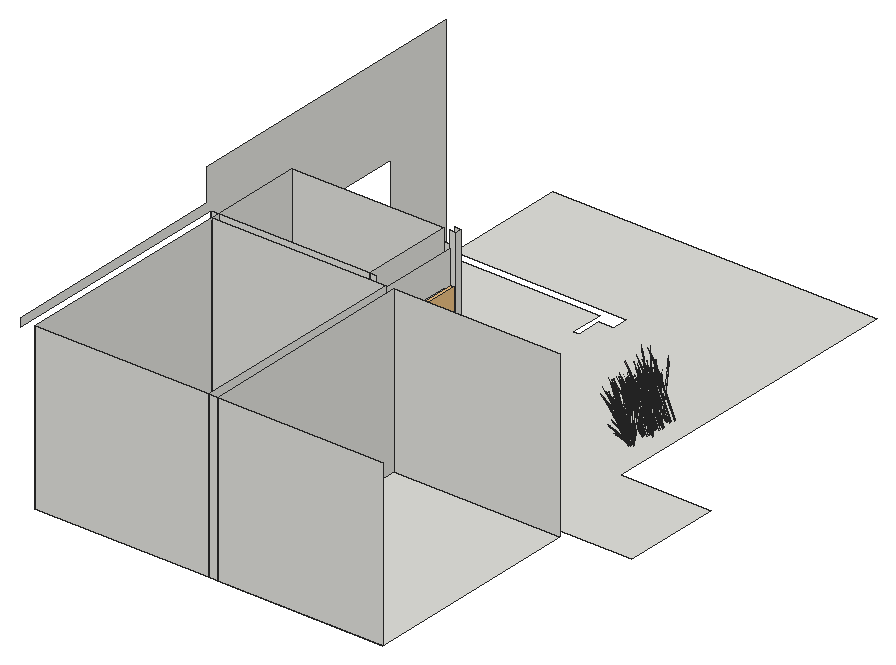
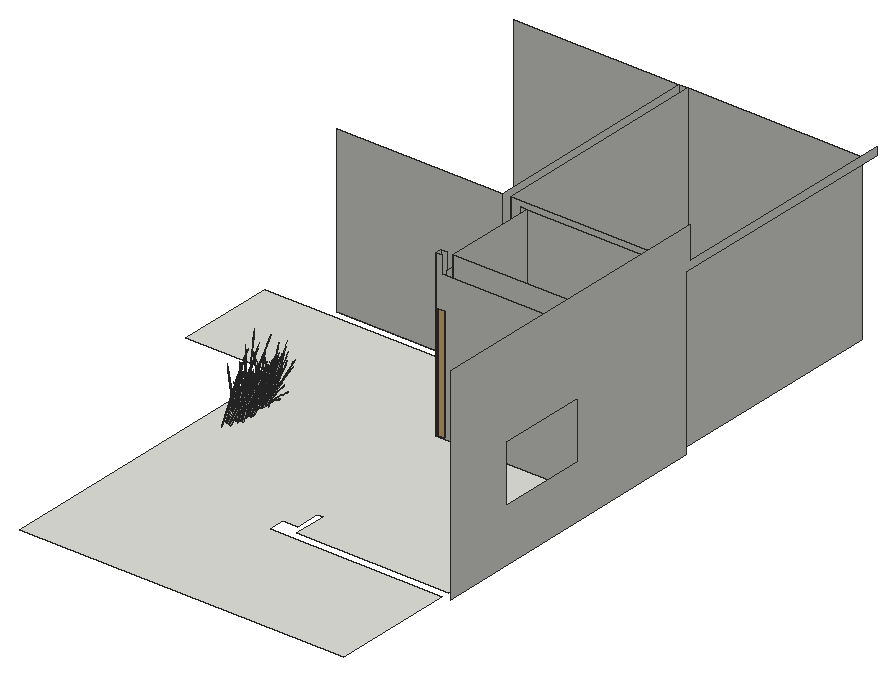
# SketchUp Ruby script. Lengths in inches.
U = 1.inch
M = Sketchup.active_model
def pt(a) = Geom::Point3d.new(a.map { |v| v * U })
def face(e, loops, mat)
  f = e.add_face(loops[0].map { |a| pt(a) })
  loops[1..].each { |l| e.add_face(l.map { |a| pt(a) }).erase! }
  f.material = f.back_material = mat if mat
  f
end
# faces: each face lists its corners as indices into pts; further lists are holes
def faces(e, pts, list, mat = nil) = list.each { |f| face(e, (f[0].is_a?(Array) ? f : [f]).map { |l| l.map { |i| pts[i] } }, mat) }
# xy, xz, yz: faces in a plane at the given z, y or x. An outline is a flat list of corners, or four numbers for a rectangle; further outlines are holes
def ring(l) = l.size == 4 ? [[l[0], l[1]], [l[2], l[1]], [l[2], l[3]], [l[0], l[3]]] : l.each_slice(2).to_a
def flat(e, list, mat, &to3) = list.each { |f| face(e, (f[0].is_a?(Array) ? f : [f]).map { |l| ring(l).map { |u, v| to3.(u, v) } }, mat) }
def xy(e, z, list, mat = nil) = flat(e, list, mat) { |x, y| [x, y, z] }
def xz(e, y, list, mat = nil) = flat(e, list, mat) { |x, z| [x, y, z] }
def yz(e, x, list, mat = nil) = flat(e, list, mat) { |y, z| [x, y, z] }
def lines(e, pts, list) = list.each { |a, b| e.add_line(pt(pts[a]), pt(pts[b])) }
# prism: a flat outline (further loops are holes) pulled along v
def prism(e, loops, v, mat = nil)
  f = face(e, loops, mat); d = Geom::Vector3d.new(v.map { |x| x * U })
  f.pushpull(f.normal.samedirection?(d) ? d.length : -d.length)
end
def box(e, o, s, mat = nil) = prism(e, [[o, [o[0] + s[0], o[1], o[2]], [o[0] + s[0], o[1] + s[1], o[2]], [o[0], o[1] + s[1], o[2]]]], [0, 0, s[2]], mat)
def at(x, y, z, deg = 0) = Geom::Transformation.translation(pt([x, y, z])) * Geom::Transformation.rotation(ORIGIN, Z_AXIS, deg.degrees)
def axes(o, x, y, z) = Geom::Transformation.new([*x, 0, *y, 0, *z, 0, *pt(o).to_a, 1])
def part(name) = M.definitions.add(name)
# library, detail: a bought-in or finely detailed component or shape, given as its bounding box
def library(name, o, s) = part(name).tap { |d| box(d.entities, o, s) }
def detail(e, o, s) = box(e.add_group.entities, o, s)
def put(e, d, t, mat = nil) = e.add_instance(d, t).tap { |i| i.material = mat if mat }
def group(e, t, mat = nil) = e.add_group.tap { |g| g.transformation = t; g.material = mat if mat }.entities
root = M.entities
M.materials.add("LightPink_Translucent").color = [144, 107, 117]
M.materials["LightPink_Translucent"].alpha = 0.75
c1 = library("porta+4",[0.2,-5.42,1.33],[46.55,4.72,83.21])
c2 = part("blade")
p = [[2.15,0.21,22],[0,0.17,0],[0.09,0.45,0],[2.18,0.31,22],[2.29,0.31,22],[0.38,0.45,0],
  [2.48,0.24,33],[2.49,0.24,33],[2.48,0.22,33]]
faces(c2.entities,p,[[0,1,2,3],[4,5,2,3],[6,3,4,7],[8,0,3,6]])
c3 = part("seeds")
p = [[0.3,-0.1,1.38],[-0.01,-0.03,1.59],[-0.01,-0.03,0.03],[0.14,-0.07,-0.07],[0.29,-0.03,3],[0.15,0.01,3.11]]
faces(c3.entities,p,[[0,1,2,3],[1,0,4,5]],"LightPink_Translucent")
c4 = part("blade with seeds")
put(c4.entities,c2,at(0,0,0))
put(c4.entities,c3,axes([2.4,0.25,30.99],[1.5799,-0.05474,1.17369],[-0.12525,1.92788,0.29478],[-0.07173,-0.02425,1.56792]))
xy(root,126,[[51,51,178.5,213],[184.5,51,306,213],[166.5,219,354,219,354,291,288,291,288,525,51,525,51,435,177,435,177,423,166.5,423,166.5,405,162,405,162,429,51,429,51,291,171,291,171,286.5,166.5,286.5],[51,219,162,286.5]])
xz(root,51,[[51,126,178.5,246],[178.5,126,184.5,246],[184.5,126,306,246]])
xz(root,213,[[51,126,178.5,246],[184.5,126,306,246]])
xz(root,219,[[45,126,51,246],[51,126,162,246],[162,126,166.5,246]])
xz(root,286.5,[[51,126,162,246],[166.5,126,171,246]])
xz(root,291,[[51,126,51,234,166.5,234,166.5,246,171,246,171,126]])
yz(root,45,[[[219,126,219,246,45,246,45,252,216,252,216,276,435,276,435,126],[318,165,384,207]]])
yz(root,51,[[51,126,213,246],[213,126,219,246],[219,126,286.5,246]])
yz(root,162,[[[219,126,286.5,246],[247.5,129,277.5,207]]])
yz(root,166.5,[[219,126,244.5,126,244.5,210,280.5,210,280.5,126,286.5,126,286.5,234,219,234],[[244.5,126,280.5,210],[247.5,129,277.5,207]]])
yz(root,171,[[286.5,126,291,246]])
yz(root,178.5,[[51,126,213,246]])
yz(root,184.5,[[51,126,213,246]])
put(root,c1,at(163.74,244.3,125.48,90))
put(root,c4,axes([268.35,323.37,125.98],[0.37107,-0.01478,1.71376],[-0.24616,0.64047,0.13857],[-0.5288,-0.03961,0.73262]))
put(root,c4,axes([268.35,336.34,126.89],[0.37107,-0.01478,1.71376],[-0.24616,0.64047,0.13857],[-0.5288,-0.03961,0.73262]))
put(root,c4,axes([268.35,346.62,126.2],[0.37107,-0.01478,1.71376],[-0.24616,0.64047,0.13857],[-0.5288,-0.03961,0.73262]))
put(root,c4,axes([268.51,324.49,125.98],[0.31041,-0.13801,1.71376],[0.26133,0.63772,0.13857],[-0.48731,0.14413,0.73262]))
put(root,c4,axes([268.51,337.47,126.89],[0.31041,-0.13801,1.71376],[0.26133,0.63772,0.13857],[-0.48731,0.14413,0.73262]))
put(root,c4,axes([268.51,347.75,126.2],[0.31041,-0.13801,1.71376],[0.26133,0.63772,0.13857],[-0.48731,0.14413,0.73262]))
put(root,c4,axes([270.29,336.8,126.35],[0.25429,-0.09438,1.77064],[0.08769,0.65901,0.13857],[-0.5508,0.08745,0.63284]))
put(root,c4,axes([270.29,347.08,125.67],[0.25429,-0.09438,1.77064],[0.08769,0.65901,0.13857],[-0.5508,0.08745,0.63284]))
put(root,c4,axes([267.56,324.27,126.82],[-0.14609,0.08471,1.74944],[0.01243,0.61893,-0.27667],[-0.33486,0.08049,0.14031]))
put(root,c4,axes([267.56,347.52,127.04],[-0.14609,0.08471,1.74944],[0.01243,0.61893,-0.27667],[-0.33486,0.08049,0.14031]))
put(root,c4,axes([269.46,335.75,127.99],[-0.89428,-0.01571,-0.71045],[0.06006,-0.66153,0.08574],[-0.37886,-0.06981,1.00501]))
put(root,c4,axes([269.46,356.56,127.625],[-0.89428,-0.01571,-0.71045],[0.06006,-0.66153,0.08574],[-0.37886,-0.06981,1.00501]))
put(root,c4,axes([268.03,323.92,126.63],[-0.74348,-0.18202,-0.35414],[0.21685,-0.53102,0.4572],[-0.29933,0.04869,0.87481]))
put(root,c4,axes([268.03,336.89,127.54],[-0.74348,-0.18202,-0.35414],[0.21685,-0.53102,0.4572],[-0.29933,0.04869,0.87481]))
put(root,c4,axes([268.03,347.17,126.85],[-0.74348,-0.18202,-0.35414],[0.21685,-0.53102,0.4572],[-0.29933,0.04869,0.87481]))
put(root,c4,axes([269.05,322.34,125.98],[0.3323,0.11241,1.71376],[-0.68769,0.4716,0.13857],[-0.42861,-0.21275,0.73262]))
put(root,c4,axes([269.05,335.32,126.89],[0.3323,0.11241,1.71376],[-0.68769,0.4716,0.13857],[-0.42861,-0.21275,0.73262]))
put(root,c4,axes([269.05,345.59,126.2],[0.3323,0.11241,1.71376],[-0.68769,0.4716,0.13857],[-0.42861,-0.21275,0.73262]))
put(root,c4,axes([269.05,356.125,126.52],[0.3323,0.11241,1.71376],[-0.68769,0.4716,0.13857],[-0.42861,-0.21275,0.73262]))
put(root,c4,axes([265.93,324.9,126.82],[0.11417,0.0175,1.77383],[0.35319,0.57649,-0.16761],[-0.23371,0.15131,0.31391]))
put(root,c4,axes([265.93,348.15,127.03],[0.11417,0.0175,1.77383],[0.35319,0.57649,-0.16761],[-0.23371,0.15131,0.31391]))
put(root,c4,axes([268.54,337.16,127.69],[-0.24236,0.59349,-0.51099],[-0.83094,-0.20343,-0.3958],[-0.33455,0.05442,0.97773]))
put(root,c4,axes([269.17,335.88,127.69],[-0.6496,0.4322,-0.51099],[-0.5689,-0.45657,-0.3958],[-0.33005,-0.06576,0.97773]))
put(root,c4,axes([269.17,356.69,127.33],[-0.6496,0.4322,-0.51099],[-0.5689,-0.45657,-0.3958],[-0.33005,-0.06576,0.97773]))
put(root,c4,axes([268.25,321.69,126.82],[0.06632,0.06511,1.77383],[-0.31973,0.58531,-0.16761],[-0.32381,0.00424,0.31391]))
put(root,c4,axes([268.25,344.95,127.03],[0.06632,0.06511,1.77383],[-0.31973,0.58531,-0.16761],[-0.32381,0.00424,0.31391]))
put(root,c4,axes([266.89,339.7,125.78],[0.37283,-0.29571,1.1486],[0.14711,0.46813,0.84392],[-0.26943,0.08382,0.25299]))
put(root,c4,axes([268.99,321.3,126.82],[-0.19249,-0.00461,1.74944],[-0.61281,0.46055,-0.27667],[-0.32697,-0.0941,0.14031]))
put(root,c4,axes([268.99,344.56,127.04],[-0.19249,-0.00461,1.74944],[-0.61281,0.46055,-0.27667],[-0.32697,-0.0941,0.14031]))
put(root,c4,axes([268.2,323.85,126.84],[0.25275,-0.59491,0.48003],[0.83094,0.20343,0.3958],[-0.32677,0.03575,0.9933]))
put(root,c4,axes([268.5,323.68,127.14],[0.45012,0.59081,-0.1216],[-0.79888,0.29033,-0.67495],[-0.33665,0.07795,1.02557]))
put(root,c4,axes([268.5,346.93,127.36],[0.45012,0.59081,-0.1216],[-0.79888,0.29033,-0.67495],[-0.33665,0.07795,1.02557]))
put(root,c4,axes([269.51,322.45,127.14],[-0.0479,0.66354,-0.1216],[-0.90696,-0.01814,-0.67495],[-0.3493,-0.04609,1.02557]))
put(root,c4,axes([269.51,345.7,127.36],[-0.0479,0.66354,-0.1216],[-0.90696,-0.01814,-0.67495],[-0.3493,-0.04609,1.02557]))
put(root,c4,axes([268.92,322.5,126.63],[-0.50902,-0.40851,-0.35414],[0.58122,-0.38671,0.4572],[-0.29531,-0.05884,0.87481]))
put(root,c4,axes([268.92,335.48,127.54],[-0.50902,-0.40851,-0.35414],[0.58122,-0.38671,0.4572],[-0.29531,-0.05884,0.87481]))
put(root,c4,axes([268.92,345.75,126.85],[-0.50902,-0.40851,-0.35414],[0.58122,-0.38671,0.4572],[-0.29531,-0.05884,0.87481]))
put(root,c4,axes([268.92,356.29,127.17],[-0.50902,-0.40851,-0.35414],[0.58122,-0.38671,0.4572],[-0.29531,-0.05884,0.87481]))
put(root,c4,axes([268.14,323.69,126.84],[-0.32857,-0.44488,0.0643],[0.59916,-0.21775,0.50621],[-0.26412,0.04296,0.77189]))
put(root,c4,axes([268.14,346.95,127.05],[-0.32857,-0.44488,0.0643],[0.59916,-0.21775,0.50621],[-0.26412,0.04296,0.77189]))
put(root,c4,axes([269.64,324.92,125.98],[0.22344,-0.20048,1.71376],[0.56419,0.54113,0.13857],[-0.38697,0.24643,0.73262]))
put(root,c4,axes([269.64,337.9,126.89],[0.22344,-0.20048,1.71376],[0.56419,0.54113,0.13857],[-0.38697,0.24643,0.73262]))
put(root,c4,axes([269.64,348.18,126.2],[0.22344,-0.20048,1.71376],[0.56419,0.54113,0.13857],[-0.38697,0.24643,0.73262]))
put(root,c4,axes([268.3,325.45,126.63],[-0.77872,0.09325,-0.35414],[-0.20563,-0.53305,0.4572],[-0.22316,0.14318,0.87481]))
put(root,c4,axes([268.3,338.42,127.54],[-0.77872,0.09325,-0.35414],[-0.20563,-0.53305,0.4572],[-0.22316,0.14318,0.87481]))
put(root,c4,axes([268.3,348.7,126.85],[-0.77872,0.09325,-0.35414],[-0.20563,-0.53305,0.4572],[-0.22316,0.14318,0.87481]))
put(root,c4,axes([267.7,336.45,125.78],[0.57115,-0.04669,1.1486],[-0.36229,0.41137,0.84392],[-0.28224,-0.06171,0.25299]))
put(root,c4,axes([268.4,325.33,126.84],[-0.22187,-0.60049,0.48003],[0.87033,-0.10422,0.3958],[-0.25651,0.14123,0.9933]))
put(root,c4,axes([268.4,348.58,127.06],[-0.22187,-0.60049,0.48003],[0.87033,-0.10422,0.3958],[-0.25651,0.14123,0.9933]))
put(root,c4,axes([268.23,325.22,126.84],[-0.61415,-0.2744,0.0643],[0.35756,-0.39076,0.50621],[-0.1969,0.12633,0.77189]))
put(root,c4,axes([268.23,348.47,127.05],[-0.61415,-0.2744,0.0643],[0.35756,-0.39076,0.50621],[-0.1969,0.12633,0.77189]))
put(root,c4,axes([269.48,325.42,125.98],[0.16657,-0.22426,1.71376],[0.69879,0.4641,0.13857],[-0.31524,0.28926,0.73262]))
put(root,c4,axes([269.48,338.39,126.89],[0.16657,-0.22426,1.71376],[0.69879,0.4641,0.13857],[-0.31524,0.28926,0.73262]))
put(root,c4,axes([269.48,348.67,126.2],[0.16657,-0.22426,1.71376],[0.69879,0.4641,0.13857],[-0.31524,0.28926,0.73262]))
put(root,c4,axes([268.81,323.86,127.16],[0.74348,0.18202,0.35414],[-0.21685,0.53102,-0.4572],[-0.29933,0.04869,0.87481]))
put(root,c4,axes([268.94,338.49,127.69],[0.22982,0.59576,-0.51099],[-0.87033,0.10422,-0.3958],[-0.24941,0.16002,0.97773]))
put(root,c4,axes([269.19,322.34,126.84],[0.04505,-0.49615,0.0643],[0.68022,0.0136,0.50621],[-0.26056,-0.05192,0.77189]))
put(root,c4,axes([269.19,345.59,127.05],[0.04505,-0.49615,0.0643],[0.68022,0.0136,0.50621],[-0.26056,-0.05192,0.77189]))
put(root,c4,axes([267.58,326.58,126.82],[-0.02224,0.12912,1.74944],[0.63107,0.44917,-0.27667],[-0.16521,0.21241,0.14031]))
put(root,c4,axes([267.58,349.83,127.04],[-0.02224,0.12912,1.74944],[0.63107,0.44917,-0.27667],[-0.16521,0.21241,0.14031]))
put(root,c4,axes([271.28,321.48,127.54],[-0.59706,0.6255,-0.13619],[-0.86465,-0.36036,-0.75594],[-0.30056,-0.17672,1.14864]))
put(root,c4,axes([271.28,344.74,127.75],[-0.59706,0.6255,-0.13619],[-0.86465,-0.36036,-0.75594],[-0.30056,-0.17672,1.14864]))
put(root,c4,axes([269.65,322.71,127.16],[0.50902,0.40851,0.35414],[-0.58122,0.38671,-0.4572],[-0.29531,-0.05884,0.87481]))
put(root,c4,axes([271.02,334.97,127.99],[-0.76283,-0.31537,-0.71045],[0.54213,-0.55263,0.08574],[-0.27638,-0.1883,1.00501]))
put(root,c4,axes([271.02,355.78,127.625],[-0.76283,-0.31537,-0.71045],[0.54213,-0.55263,0.08574],[-0.27638,-0.1883,1.00501]))
put(root,c4,axes([270.66,334.98,127.69],[-0.88277,0.1551,-0.51099],[-0.15442,-0.58737,-0.3958],[-0.23711,-0.16832,0.97773]))
put(root,c4,axes([270.66,355.79,127.33],[-0.88277,0.1551,-0.51099],[-0.15442,-0.58737,-0.3958],[-0.23711,-0.16832,0.97773]))
put(root,c4,axes([268.53,325.08,127.14],[0.82753,0.35977,-0.1216],[-0.47675,0.52101,-0.67495],[-0.2338,0.18111,1.02557]))
put(root,c4,axes([268.53,348.34,127.36],[0.82753,0.35977,-0.1216],[-0.47675,0.52101,-0.67495],[-0.2338,0.18111,1.02557]))
put(root,c4,axes([268.93,325.13,127.16],[0.77872,-0.09325,0.35414],[0.20563,0.53305,-0.4572],[-0.22316,0.14318,0.87481]))
put(root,c4,axes([271.05,320,126.82],[-0.01669,0.07821,1.77383],[-0.82314,0.28383,-0.16761],[-0.24223,-0.14508,0.31391]))
put(root,c4,axes([271.05,343.25,127.03],[-0.01669,0.07821,1.77383],[-0.82314,0.28383,-0.16761],[-0.24223,-0.14508,0.31391]))
put(root,c4,axes([270.42,321.68,125.98],[0.2045,0.20949,1.71376],[-0.94495,0.17636,0.13857],[-0.21357,-0.32887,0.73262]))
put(root,c4,axes([270.42,334.66,126.89],[0.2045,0.20949,1.71376],[-0.94495,0.17636,0.13857],[-0.21357,-0.32887,0.73262]))
put(root,c4,axes([270.42,344.9375,126.2],[0.2045,0.20949,1.71376],[-0.94495,0.17636,0.13857],[-0.21357,-0.32887,0.73262]))
put(root,c4,axes([270.42,355.47,126.52],[0.2045,0.20949,1.71376],[-0.94495,0.17636,0.13857],[-0.21357,-0.32887,0.73262]))
put(root,c4,axes([269.67,326.55,126.84],[-0.63704,-0.44518,0.48003],[0.67652,-0.38394,0.3958],[-0.11751,0.20886,0.9933]))
put(root,c4,axes([270.75,321.57,126.63],[-0.13817,-0.52554,-0.35414],[0.78985,-0.13877,0.4572],[-0.21215,-0.1506,0.87481]))
put(root,c4,axes([270.75,334.55,127.54],[-0.13817,-0.52554,-0.35414],[0.78985,-0.13877,0.4572],[-0.21215,-0.1506,0.87481]))
put(root,c4,axes([270.75,344.83,126.85],[-0.13817,-0.52554,-0.35414],[0.78985,-0.13877,0.4572],[-0.21215,-0.1506,0.87481]))
put(root,c4,axes([270.75,355.36,127.17],[-0.13817,-0.52554,-0.35414],[0.78985,-0.13877,0.4572],[-0.21215,-0.1506,0.87481]))
put(root,c4,axes([269.4375,326.51,126.84],[-0.73517,-0.0304,0.0643],[0.02016,-0.45906,0.50621],[-0.07693,0.17585,0.77189]))
put(root,c4,axes([269.4375,349.76,127.05],[-0.73517,-0.0304,0.0643],[0.02016,-0.45906,0.50621],[-0.07693,0.17585,0.77189]))
put(root,c4,axes([269.67,326.68,126.63],[-0.60531,0.34352,-0.35414],[-0.573,-0.39225,0.4572],[-0.08718,0.19929,0.87481]))
put(root,c4,axes([269.67,339.66,127.54],[-0.60531,0.34352,-0.35414],[-0.573,-0.39225,0.4572],[-0.08718,0.19929,0.87481]))
put(root,c4,axes([269.67,349.93,126.85],[-0.60531,0.34352,-0.35414],[-0.573,-0.39225,0.4572],[-0.08718,0.19929,0.87481]))
put(root,c4,axes([271.22,322,127.16],[0.13817,0.52554,0.35414],[-0.78985,0.13877,-0.4572],[-0.21215,-0.1506,0.87481]))
put(root,c4,axes([267.51,327.9,126.82],[0.10149,-0.03939,1.77383],[0.83886,0.26202,-0.16761],[-0.01971,0.21816,0.31391]))
put(root,c4,axes([267.51,351.16,127.03],[0.10149,-0.03939,1.77383],[0.83886,0.26202,-0.16761],[-0.01971,0.21816,0.31391]))
put(root,c4,axes([272.84,338.54,126.34],[0.77308,0.2631,1.51261],[-0.75736,0.56681,0.59816],[-0.33924,-0.33594,1.26806]))
put(root,c4,axes([272.84,348.8125,125.65],[0.77308,0.2631,1.51261],[-0.75736,0.56681,0.59816],[-0.33924,-0.33594,1.26806]))
put(root,c4,axes([272.84,359.35,125.97],[0.77308,0.2631,1.51261],[-0.75736,0.56681,0.59816],[-0.33924,-0.33594,1.26806]))
put(root,c4,axes([269.89,333.76,125.78],[0.46666,0.22709,1.1486],[-0.67962,0.13651,0.84392],[-0.14541,-0.17452,0.25299]))
put(root,c4,axes([270.07,339.3,128.35],[-0.02328,0.60353,-0.7886],[-0.98022,-0.04053,0.09517],[-0.10344,0.25568,1.11556]))
put(root,c4,axes([270.05,340.99,125.78],[-0.02315,-0.38796,1.1486],[0.57853,0.27671,0.84392],[-0.11378,0.18492,0.25299]))
put(root,c4,axes([271.09,321.53,126.84],[0.4066,-0.41448,0.0643],[0.57901,0.24131,0.50621],[-0.18719,-0.13288,0.77189]))
put(root,c4,axes([271.09,344.78,127.05],[0.4066,-0.41448,0.0643],[0.57901,0.24131,0.50621],[-0.18719,-0.13288,0.77189]))
put(root,c4,axes([270.88,339.36,125.49],[0.83726,0.32623,0.49651],[-0.50045,0.58498,0],[-0.19069,-0.0743,1.57504]))
put(root,c4,axes([269.74,340.15,126.375],[0.01966,-0.33682,1.54345],[0.88405,0.17791,0.21329],[-0.0766,0.35897,0.72882]))
put(root,c4,axes([271.98,320.3,126.82],[-0.13683,-0.09148,1.74944],[-0.91315,0.058,-0.27667],[-0.14574,-0.2188,0.14031]))
put(root,c4,axes([271.98,343.55,127.04],[-0.13683,-0.09148,1.74944],[-0.91315,0.058,-0.27667],[-0.14574,-0.2188,0.14031]))
put(root,c4,axes([270.27,339.5,128.02],[0.64041,0.4384,-0.5672],[-0.67652,0.38394,-0.43934],[-0.09744,0.22274,1.08528]))
put(root,c4,axes([270.27,349.77,127.33],[0.64041,0.4384,-0.5672],[-0.67652,0.38394,-0.43934],[-0.09744,0.22274,1.08528]))
put(root,c4,axes([269.98,326.19,127.16],[0.60531,-0.34352,0.35414],[0.573,0.39225,-0.4572],[-0.08718,0.19929,0.87481]))
put(root,c4,axes([274.04,337.28,125.85],[-0.02444,-0.61432,1.41272],[1.10603,0.15924,0.59816],[-0.26159,0.33615,1.3335]))
put(root,c4,axes([269.6,326.29,127.5],[0.98321,0.03233,-0.13498],[-0.02687,0.61208,-0.74919],[-0.0683,0.23574,1.13838]))
put(root,c4,axes([269.6,349.54,127.72],[0.98321,0.03233,-0.13498],[-0.02687,0.61208,-0.74919],[-0.0683,0.23574,1.13838]))
put(root,c4,axes([273.37,321.71,127.14],[-0.87543,0.30377,-0.1216],[-0.4302,-0.53915,-0.67495],[-0.1155,-0.2272,1.02557]))
put(root,c4,axes([273.37,344.96,127.36],[-0.87543,0.30377,-0.1216],[-0.4302,-0.53915,-0.67495],[-0.1155,-0.2272,1.02557]))
put(root,c4,axes([273.37,355.5,127.68],[-0.87543,0.30377,-0.1216],[-0.4302,-0.53915,-0.67495],[-0.1155,-0.2272,1.02557]))
put(root,c4,axes([272.62,334.71,127.69],[-0.87941,-0.16356,-0.51099],[0.30143,-0.56078,-0.3958],[-0.08064,-0.22578,0.97773]))
put(root,c4,axes([272.62,355.52,127.33],[-0.87941,-0.16356,-0.51099],[0.30143,-0.56078,-0.3958],[-0.08064,-0.22578,0.97773]))
